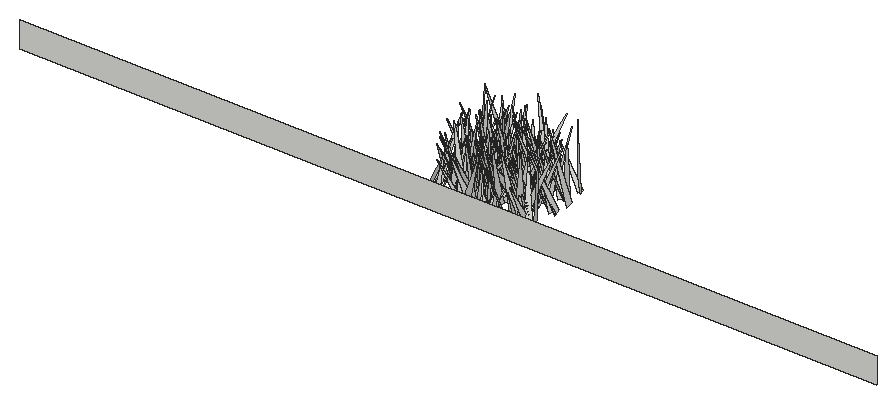
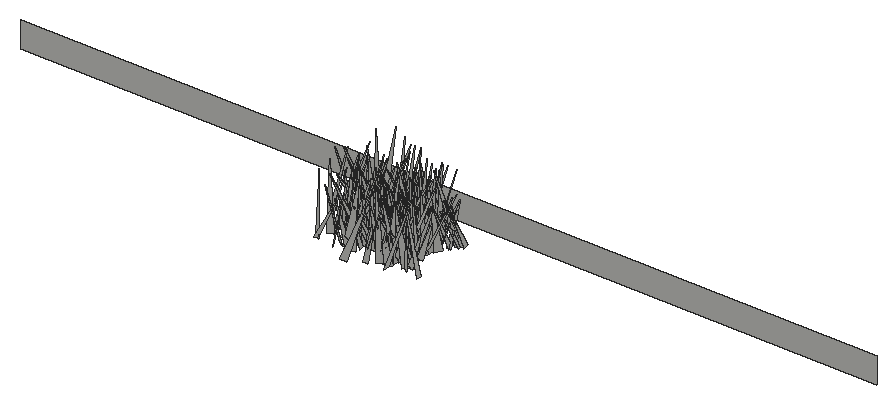
# SketchUp Ruby script. Lengths in inches.
U = 1.inch
M = Sketchup.active_model
def pt(a) = Geom::Point3d.new(a.map { |v| v * U })
def face(e, loops, mat)
  f = e.add_face(loops[0].map { |a| pt(a) })
  loops[1..].each { |l| e.add_face(l.map { |a| pt(a) }).erase! }
  f.material = f.back_material = mat if mat
  f
end
# faces: each face lists its corners as indices into pts; further lists are holes
def faces(e, pts, list, mat = nil) = list.each { |f| face(e, (f[0].is_a?(Array) ? f : [f]).map { |l| l.map { |i| pts[i] } }, mat) }
# xy, xz, yz: faces in a plane at the given z, y or x. An outline is a flat list of corners, or four numbers for a rectangle; further outlines are holes
def ring(l) = l.size == 4 ? [[l[0], l[1]], [l[2], l[1]], [l[2], l[3]], [l[0], l[3]]] : l.each_slice(2).to_a
def flat(e, list, mat, &to3) = list.each { |f| face(e, (f[0].is_a?(Array) ? f : [f]).map { |l| ring(l).map { |u, v| to3.(u, v) } }, mat) }
def xy(e, z, list, mat = nil) = flat(e, list, mat) { |x, y| [x, y, z] }
def xz(e, y, list, mat = nil) = flat(e, list, mat) { |x, z| [x, y, z] }
def yz(e, x, list, mat = nil) = flat(e, list, mat) { |y, z| [x, y, z] }
def lines(e, pts, list) = list.each { |a, b| e.add_line(pt(pts[a]), pt(pts[b])) }
# prism: a flat outline (further loops are holes) pulled along v
def prism(e, loops, v, mat = nil)
  f = face(e, loops, mat); d = Geom::Vector3d.new(v.map { |x| x * U })
  f.pushpull(f.normal.samedirection?(d) ? d.length : -d.length)
end
def box(e, o, s, mat = nil) = prism(e, [[o, [o[0] + s[0], o[1], o[2]], [o[0] + s[0], o[1] + s[1], o[2]], [o[0], o[1] + s[1], o[2]]]], [0, 0, s[2]], mat)
def at(x, y, z, deg = 0) = Geom::Transformation.translation(pt([x, y, z])) * Geom::Transformation.rotation(ORIGIN, Z_AXIS, deg.degrees)
def axes(o, x, y, z) = Geom::Transformation.new([*x, 0, *y, 0, *z, 0, *pt(o).to_a, 1])
def part(name) = M.definitions.add(name)
# library, detail: a bought-in or finely detailed component or shape, given as its bounding box
def library(name, o, s) = part(name).tap { |d| box(d.entities, o, s) }
def detail(e, o, s) = box(e.add_group.entities, o, s)
def put(e, d, t, mat = nil) = e.add_instance(d, t).tap { |i| i.material = mat if mat }
def group(e, t, mat = nil) = e.add_group.tap { |g| g.transformation = t; g.material = mat if mat }.entities
root = M.entities
c1 = part("fur_instance\#9")
p = [[0.8125,0,1.79],[0.67,-0.02,1.48],[0,-0.11,0],[0,0.11,0]]
faces(c1.entities,p,[[0,1,2,3]])
xz(root,5.77,[[0,-27.625,196.6875,-21.625]])
put(root,c1,axes([98.54,11.75,-27.1],[2.87814,-5.28951,1.31735],[-4.95416,-3.15966,-1.86304],[-2.27391,0.18887,5.72641]))
put(root,c1,axes([108.72,12.08,-27.1],[6.46231,-4.31648,2.52967],[-3.92803,-6.93665,-1.8017],[-3.09867,-0.20881,7.55958]))
put(root,c1,axes([97.8,11.71,-27.1],[2.89446,-5.47209,0.08006],[-5.31049,-2.7865,1.53693],[1.32243,0.78724,5.99662]))
put(root,c1,axes([108.44,12.38,-27.1],[4.1039,-1.37964,0.4984],[-1.03776,-3.77714,-1.91052],[-1.03675,-1.68037,3.88527]))
put(root,c1,axes([97.1,14.13,-27.1],[5.11337,-4.37567,0.02712],[-4.08728,-4.79107,-2.37351],[-1.56248,-1.78687,6.29758]))
put(root,c1,axes([110.18,13.09,-27.1],[4.14247,-2.36814,0.94959],[-1.79033,-3.98803,-2.13546],[-1.81783,-1.46881,4.26707]))
put(root,c1,axes([100.52,11.44,-27.1],[3.76138,-1.24538,0.93866],[-1.27843,-3.86595,-0.00634],[-0.89313,0.28885,3.96218]))
put(root,c1,axes([94.32,12.76,-27.1],[-3.93279,-0.23592,0.50656],[-0.05149,3.7386,1.34138],[0.55643,-1.32147,3.70448]))
put(root,c1,axes([99.45,11.81,-27.1],[1.25077,5.74635,3.18749],[6.40163,-1.79789,0.7292],[-1.48314,-2.91412,5.83551]))
put(root,c1,axes([99.67,13.3,-27.1],[6.5233,2.37968,3.04495],[3.30026,-6.53866,-1.96019],[-2.01069,-3.01183,6.66138]))
put(root,c1,axes([103.65,14.05,-27.1],[7.48346,-2.4752,1.75576],[-1.96533,-7.51292,-2.21472],[-2.31232,-1.62508,7.56464]))
put(root,c1,axes([104.87,12.96,-27.1],[-1.89303,-4.40404,0.51291],[-4.43222,1.86471,-0.34716],[-0.11875,0.60786,4.78107]))
put(root,c1,axes([103.4,14.22,-27.1],[-5.97447,-2.65496,2.2585],[-2.10106,6.3191,1.8704],[2.78122,-0.92951,6.26456]))
put(root,c1,axes([107.73,14.55,-27.1],[5.80631,-5.6916,0.53269],[-5.68589,-5.82856,-0.29992],[-0.59055,0.15799,8.12513]))
put(root,c1,axes([103.21,11.5,-27.1],[-0.85161,3.55792,0.87868],[3.50079,1.05663,-0.88551],[1.08413,-0.61714,3.54963]))
put(root,c1,axes([103.73,12.08,-27.1],[3.9323,-0.29865,1.47953],[-0.48436,-4.16008,0.44758],[-1.42954,0.58799,3.91814]))
put(root,c1,axes([96.6,12.32,-27.1],[5.34271,-3.44394,4.19103],[-3.85612,-6.54857,-0.46545],[-3.8152,1.796,6.33945]))
put(root,c1,axes([100.63,11.89,-27.1],[-2.63101,2.88231,1.12737],[2.88894,2.81797,-0.46255],[1.11028,-0.50218,3.87505]))
put(root,c1,axes([101.61,15.49,-27.1],[-1.56855,-7.63886,0.47282],[-7.63369,1.59619,0.46371],[0.55001,0.36889,7.78444]))
put(root,c1,axes([101.04,15.37,-27.1],[-1.24529,-7.71146,0.7872],[-7.61167,1.36728,1.35282],[1.46589,0.54863,7.69333]))
put(root,c1,axes([103.93,12.45,-27.1],[-0.42673,3.51272,1.26133],[3.73148,0.37463,0.21911],[-0.0791,-1.27778,3.53176]))
put(root,c1,axes([93.95,15.29,-27.1],[-5.87667,-3.9224,1.1719],[-3.54254,5.90008,1.98324],[2.05159,-1.04767,6.78139]))
put(root,c1,axes([104.39,17.625,-27.1],[6.48177,-5.01878,0.45242],[-4.24735,-5.8379,-3.90962],[-2.71162,-2.85253,7.2053]))
put(root,c1,axes([90.46,12.68,-27.1],[1.50954,-3.07856,1.78204],[-3.55315,-1.39659,0.59714],[-0.16832,1.87187,3.37633]))
put(root,c1,axes([103.32,12.72,-27.1],[4.26257,2.91433,0.00484],[2.86478,-4.18851,-0.95515],[0.53516,-0.79116,5.0745]))
put(root,c1,axes([101.18,13.5,-27.1],[-4.07281,-4.5818,0.7427],[-4.55178,3.7491,-1.83244],[-0.90871,1.75604,5.85003]))
put(root,c1,axes([110.46,13.58,-27.1],[-2.82559,-5.19892,1.36333],[-5.31081,2.46391,-1.61114],[-0.82624,1.9421,5.69358]))
put(root,c1,axes([101.12,13.64,-27.1],[-2.2184,-4.85625,2.50772],[-5.03427,2.86928,1.10295],[2.1279,1.72546,5.22379]))
put(root,c1,axes([91.81,12.22,-27.1],[4.67763,2.46387,0.32375],[2.42875,-4.67875,0.51598],[-0.52599,0.30722,5.26162]))
put(root,c1,axes([96.28,12.86,-27.1],[3.51282,6.48869,2.15536],[6.79895,-3.57131,-0.32959],[-0.72316,-2.057,7.37118]))
put(root,c1,axes([101.98,16.15,-27.1],[0.91658,-6.09487,0.23316],[-5.96683,-0.94489,-1.24341],[-1.26442,0.04079,6.03668]))
put(root,c1,axes([112.29,13.32,-27.1],[-4.83531,-1.63891,2.39644],[-2.01972,5.24312,-0.48946],[2.08559,1.27782,5.08199]))
put(root,c1,axes([93.04,14.27,-27.1],[-5.61419,2.77509,3.47904],[3.15086,6.4338,-0.04739],[3.14276,-1.49299,6.26243]))
put(root,c1,axes([94.93,15.09,-27.1],[-3.76268,-4.24685,0.11424],[-4.17448,3.66755,-1.15295],[-0.78896,0.84846,5.55555]))
put(root,c1,axes([88.44,13.02,-27.1],[5.14686,-0.10254,0.48257],[-0.21946,-5.00543,1.27711],[-0.44184,1.29176,4.98695]))
put(root,c1,axes([90.48,15.46,-27.1],[-0.08561,-4.51883,0.61864],[-4.55746,0.06047,-0.18896],[-0.17898,0.62161,4.51569]))
put(root,c1,axes([100.42,13.8125,-27.1],[-4.38445,3.57185,1.79964],[3.76738,4.58485,0.07863],[1.34299,-1.20052,5.65467]))
put(root,c1,axes([109.75,12.12,-27.1],[-6.16922,0.32467,1.04524],[-0.06119,5.87189,-2.18505],[1.09279,2.16166,5.77844]))
put(root,c1,axes([100.8125,13.96,-27.1],[-6.07164,-2.28107,2.04855],[-2.55827,6.27412,-0.5961],[1.68971,1.3026,6.45854]))
put(root,c1,axes([98.98,15.98,-27.1],[-1.13114,-4.608,0.05517],[-4.59723,1.12439,-0.34274],[-0.31976,0.13515,4.73241]))
put(root,c1,axes([98.36,14.21,-27.1],[4.34126,2.62004,0.01209],[2.52851,-4.18338,-1.34808],[0.68659,-1.1602,4.88813]))
put(root,c1,axes([98.34,13.66,-27.1],[4.70359,-4.43483,0.77561],[-4.1988,-3.91632,3.07011],[1.62462,2.71804,5.6891]))
put(root,c1,axes([110.84,12.96,-27.1],[-3.10471,5.12305,0.88051],[5.18598,3.12286,0.11631],[0.35573,-0.81381,5.98927]))
put(root,c1,axes([97.03,15.39,-27.1],[-4.89402,-3.33819,1.83703],[-3.30827,5.20635,0.64726],[1.89038,0.46913,5.88863]))
put(root,c1,axes([108.12,16.37,-27.1],[-3.94207,-4.94022,1.13908],[-4.81769,4.09962,1.10733],[1.57897,0.1748,6.2225]))
put(root,c1,axes([93.34,14.85,-27.1],[3.78435,-1.32179,0.68035],[-1.35222,-3.83372,0.07338],[-0.61764,0.29457,4.00787]))
put(root,c1,axes([100.32,14.03,-27.1],[-1.02594,6.32348,2.52203],[6.58274,1.57191,-1.26344],[1.73626,-2.22313,6.28034]))
put(root,c1,axes([99.11,15.625,-27.1],[1.24719,-3.91493,0.4967],[-3.8954,-1.13791,0.81231],[0.63182,0.71228,4.02769]))
put(root,c1,axes([100.35,15.59,-27.1],[-1.33091,-4.34516,1.37723],[-4.35803,1.6335,0.94222],[1.33595,0.99989,4.44566]))
put(root,c1,axes([93.37,14.92,-27.1],[0.69074,-4.72184,2.34998],[-4.89788,-1.45354,-1.48096],[-1.95676,1.97148,4.53648]))
put(root,c1,axes([89.04,13.88,-27.1],[4.0967,-0.1052,0.02727],[-0.10864,-3.93802,1.12914],[0.00278,1.12946,3.93942]))
put(root,c1,axes([94.33,14.38,-27.1],[-2.33068,3.85921,0.35584],[3.66264,2.05758,1.6744],[-1.26695,-1.15111,4.18592]))
put(root,c1,axes([89.42,13.98,-27.1],[0.24663,7.62872,2.41582],[7.70784,0.42293,-2.12242],[2.15005,-2.39126,7.33168]))
put(root,c1,axes([104.46,16.01,-27.1],[-2.38494,-6.16406,1.52656],[-6.35023,2.30898,-0.59758],[-0.0234,1.63919,6.58229]))
put(root,c1,axes([108.95,14.06,-27.1],[5.79439,-3.93356,1.43708],[-4.17619,-5.2444,2.48372],[0.31237,2.85246,6.54821]))
put(root,c1,axes([92.67,14.32,-27.1],[-3.84784,-1.19504,0.32807],[-1.23606,3.62421,-1.29571],[-0.08892,1.33363,3.81512]))
put(root,c1,axes([106.33,16.25,-27.1],[-3.36385,-0.86607,1.07357],[-0.51946,3.41676,1.12873],[1.27781,-0.89095,3.28504]))
put(root,c1,axes([103.16,15.92,-27.1],[-3.34237,-3.67886,0.49489],[-3.71061,3.29315,-0.58039],[-0.10119,0.75599,4.93646]))
put(root,c1,axes([91.96,16.72,-27.1],[-3.17916,-2.57933,0.00353],[-2.53731,3.12837,0.73174],[0.46373,-0.56605,4.02798]))
put(root,c1,axes([105.08,15.55,-27.1],[-3.3946,-3.12525,1.18102],[-3.29173,3.41661,-0.4203],[0.5714,1.11577,4.59499]))
put(root,c1,axes([105.97,17.65,-27.1],[2.24091,-5.47361,0.67385],[-5.23088,-2.33999,-1.61199],[-1.7471,-0.01469,5.69066]))
put(root,c1,axes([98.25,15.02,-27.1],[4.49912,0.07902,0.02983],[0.07502,-4.46879,0.52292],[-0.03881,0.52233,4.46932]))
put(root,c1,axes([97.99,16.47,-27.1],[1.8485,-3.49978,1.33816],[-3.45042,-2.17169,-0.91344],[-1.46071,0.70098,3.8511]))
put(root,c1,axes([110.15,19.25,-27.1],[-3.50557,-5.51536,0.11612],[-4.95597,3.20905,2.80393],[2.42302,-1.41579,5.90306]))
put(root,c1,axes([106.26,16.66,-27.1],[2.2039,-6.87435,1.74953],[-7.02125,-1.85328,1.56272],[1.00974,2.1174,7.04782]))
put(root,c1,axes([103.87,15.71,-27.1],[-0.77186,4.35622,1.72795],[4.2436,-0.09339,2.13104],[-1.98854,-1.8902,3.87699]))
put(root,c1,axes([113.22,18.26,-27.1],[-7.42684,-1.75978,1.28146],[-1.36577,7.3143,2.12899],[1.69519,-1.81689,7.32954]))
put(root,c1,axes([109.69,16.92,-27.1],[-5.35424,-1.86738,0.02315],[-1.86377,5.3475,0.29345],[0.11847,-0.26947,5.66294]))
put(root,c1,axes([95.07,18.68,-27.1],[7.37439,-3.31849,1.28024],[-2.90244,-7.31769,-2.24953],[-2.05603,-1.57231,7.76747]))
put(root,c1,axes([102.41,13.9,-27.1],[0.90469,6.24799,0.05202],[5.52251,-0.775,-2.9597],[2.92267,-0.46962,5.57638]))
put(root,c1,axes([95.3,13.15,-27.1],[-7.34828,2.49323,1.09592],[2.03506,7.1224,-2.5582],[1.80991,2.11416,7.32591]))
put(root,c1,axes([97.38,17.34,-27.1],[2.10827,-4.41232,0.88185],[-4.4927,-2.11805,0.1432],[-0.24874,0.85808,4.88803]))
put(root,c1,axes([101.06,16,-27.1],[1.63148,3.88333,0.8996],[3.80186,-1.22375,-1.61232],[1.19808,-1.40479,3.89132]))
put(root,c1,axes([107.17,18.27,-27.1],[1.92624,-6.27783,0.49509],[-6.26935,-1.863,0.76884],[0.59288,0.69623,6.52153]))
put(root,c1,axes([101.15,19.08,-27.1],[5.45875,-2.61976,0.1584],[-2.41646,-5.15945,-2.05595],[-1.02417,-1.78972,5.6951]))
put(root,c1,axes([104.25,19.42,-27.1],[-5.79035,-4.99721,0.36352],[-4.82955,5.71454,1.62848],[1.33407,-1.00217,7.47317]))
put(root,c1,axes([93.13,18.07,-27.1],[2.46891,-7.20313,1.70316],[-7.36136,-2.57683,-0.22704],[-0.77207,1.53499,7.61111]))
put(root,c1,axes([92.8,15.74,-27.1],[3.62084,3.81527,1.03017],[3.87963,-3.69771,0.05854],[-0.75237,-0.70613,5.25959]))
put(root,c1,axes([105.57,16.87,-27.1],[3.73995,-4.97965,1.07609],[-4.97131,-3.27521,2.12161],[1.114,2.10195,5.85517]))
put(root,c1,axes([90.45,15.07,-27.1],[4.99403,0.89918,1.35491],[0.3935,-4.91429,1.81096],[-1.5778,1.62046,4.74018]))
put(root,c1,axes([95.3125,15.46,-27.1],[4.61387,-2.10989,0.31356],[-1.93342,-3.82099,2.73855],[0.90102,2.60502,4.2708]))
put(root,c1,axes([96.03,16.4,-27.1],[3.36091,-1.13304,0.9234],[-1.35023,-3.29337,0.87337],[-0.55977,1.1411,3.43755]))
put(root,c1,axes([94.78,18.22,-27.1],[-2.52034,-4.28654,0.32351],[-4.12689,2.30776,-1.57296],[-1.20326,1.06349,4.71724]))
put(root,c1,axes([113.24,18.05,-27.1],[-6.30191,-3.29477,0.26908],[-3.30318,6.25333,-0.79169],[-0.13009,0.82599,7.06702]))
put(root,c1,axes([98.65,18.3125,-27.1],[-4.19066,-2.50752,1.09961],[-2.47633,4.32875,0.43379],[1.16817,0.18082,4.86427]))
put(root,c1,axes([112.28,17.91,-27.1],[-4.9541,1.83691,1.27432],[2.05779,4.95762,0.85363],[0.87385,-1.26054,5.21428]))
put(root,c1,axes([102.53,14.22,-27.1],[3.62911,6.60842,0.2466],[6.35712,-3.56375,1.94657],[-1.82181,0.72867,7.28371]))
put(root,c1,axes([91.14,17.54,-27.1],[5.12672,-4.5376,2.59386],[-5.0883,-5.16347,1.02416],[-1.19461,2.5199,6.76936]))
put(root,c1,axes([98.95,19.43,-27.1],[-3.68425,-5.36529,0.32526],[-5.32374,3.58793,-1.11818],[-0.74155,0.8979,6.41168]))
put(root,c1,axes([103.25,18.7,-27.1],[-1.22069,-3.41408,1.05948],[-3.55821,1.26785,-0.01408],[0.34288,1.00256,3.62571]))
put(root,c1,axes([99.66,18.9375,-27.1],[-3.20699,2.34244,2.63387],[2.95903,3.72406,0.29089],[1.91533,-1.83124,3.96071]))
put(root,c1,axes([108.55,18.625,-27.1],[4.54413,5.8348,1.67226],[5.93472,-3.83302,-2.75273],[1.27295,-2.95864,6.86415]))
put(root,c1,axes([103.3125,18.64,-27.1],[-0.92871,-3.83483,1.6083],[-4.04735,1.2119,0.55253],[0.95473,1.40727,3.90681]))
put(root,c1,axes([96.76,18.89,-27.1],[0.02782,-4.7345,1.86898],[-5.06027,0.17616,0.52158],[0.54982,1.86087,4.70577]))
put(root,c1,axes([108.96,19.18,-27.1],[3.6892,-1.49713,1.29137],[-1.47127,-3.90506,-0.32413],[-1.32076,0.16824,3.96818]))
put(root,c1,axes([92.43,20.0625,-27.1],[2.19919,-5.46865,1.19281],[-5.58851,-2.07385,0.79564],[0.31218,1.39943,5.84033]))
put(root,c1,axes([92.4,20.07,-27.1],[-5.87087,-0.65311,0.1721],[-0.62527,5.82501,0.77566],[0.25536,-0.75237,5.85594]))
put(root,c1,axes([104.39,17.93,-27.1],[3.12045,6.97557,0.92804],[6.87353,-2.80376,-2.03727],[1.5081,-1.6545,7.36514]))
put(root,c1,axes([110.32,14.52,-27.1],[5.94606,5.36025,0.59468],[4.2161,-5.17199,4.4628],[-3.36309,2.9933,6.64615]))
put(root,c1,axes([92,18.89,-27.1],[-5.13165,1.21269,1.54361],[1.09048,5.35359,-0.58061],[1.63224,0.23592,5.24093]))
put(root,c1,axes([106.85,20.65,-27.1],[2.3512,-5.85332,1.44977],[-6.03015,-2.28819,0.5412],[-0.02311,1.54732,6.28463]))
put(root,c1,axes([100.87,20.15,-27.1],[4.61711,2.95667,1.94744],[3.35791,-4.67134,-0.86895],[-1.12198,-1.8135,5.41336]))
put(root,c1,axes([99.21,19.03,-27.1],[-3.06534,4.86368,0.18481],[4.51167,2.75744,2.26433],[-1.82603,-1.35165,5.28436]))
put(root,c1,axes([101.11,20.35,-27.1],[4.30698,0.82715,0.77594],[0.97071,-4.26434,-0.84231],[-0.5865,-0.98365,4.30404]))
put(root,c1,axes([100.98,20.16,-27.1],[-2.4507,-4.58404,1.24543],[-4.71435,2.17524,-1.27033],[-0.58261,1.68089,5.0404]))
put(root,c1,axes([106.03,20.35,-27.1],[4.89735,3.35239,2.18214],[3.80193,-4.97328,-0.89225],[-1.24321,-2.00306,5.86741]))
put(root,c1,axes([104.77,18.31,-27.1],[1.00631,5.78428,1.17144],[5.41169,-1.37849,2.15781],[-2.35451,-0.6962,5.46025]))
put(root,c1,axes([94.97,21.88,-27.1],[-4.99858,-6.00178,0.67378],[-6.03784,4.94565,-0.739],[-0.1407,0.9901,7.77567]))
put(root,c1,axes([106.64,22.57,-27.1],[-7.7703,-1.5883,1.42664],[-1.2052,7.70803,2.01725],[1.76224,-1.7318,7.67014]))
put(root,c1,axes([93.95,20.4,-27.1],[-5.48132,1.03762,0.48302],[1.07413,5.47965,0.41785],[0.39525,-0.50168,5.563]))
put(root,c1,axes([94.95,20.97,-27.1],[5.5976,-0.64404,1.05715],[-0.59203,-5.69245,-0.3332],[-1.08713,-0.21617,5.62467]))
put(root,c1,axes([93.49,22.07,-27.1],[0.81031,-5.69395,0.84212],[-5.55553,-0.55126,1.61834],[1.50543,1.03047,5.51893]))
put(root,c1,axes([110.77,22.91,-27.1],[-3.23676,-6.95107,0.75182],[-6.9834,3.25434,0.02332],[0.33861,0.67166,7.66769]))
put(root,c1,axes([93.72,21.75,-27.1],[-0.85908,-3.57953,0.71794],[-3.54097,0.99653,0.73143],[0.88884,0.51028,3.60778]))
put(root,c1,axes([99.27,20.74,-27.1],[-4.79619,2.23097,0.90337],[2.34699,4.78153,0.65218],[0.53379,-0.97799,5.24932]))
put(root,c1,axes([113.23,21.92,-27.1],[-7.82049,-1.65264,1.82204],[-1.48703,8.01344,0.88582],[1.95953,-0.51451,7.94397]))
put(root,c1,axes([94.43,22.45,-27.1],[6.50516,0.09741,3.11354],[0.81371,-7.01185,-1.48071],[-3.00691,-1.68675,6.33514]))
put(root,c1,axes([104.8125,20.66,-27.1],[3.28542,-2.52777,1.83261],[-2.97263,-3.34603,0.71392],[-0.95477,1.71946,4.08337]))
put(root,c1,axes([93.3125,21.35,-27.1],[6.93717,-2.75986,2.51351],[-2.97128,-7.29338,0.19237],[-2.25967,1.11744,7.46352]))
put(root,c1,axes([102.1,21.9,-27.1],[1.8151,-3.86013,1.55176],[-3.9232,-2.15155,-0.76319],[-1.38458,1.03602,4.19675]))
put(root,c1,axes([100.08,19.92,-27.1],[3.50829,2.33455,0.59392],[2.17247,-3.51961,1.00185],[-1.04078,0.52272,4.09323]))
put(root,c1,axes([100.59,19.74,-27.1],[-4.5545,1.12209,0.15618],[1.0267,4.36161,-1.39615],[0.47894,1.3207,4.4781]))
put(root,c1,axes([97.65,24.4,-27.1],[7.10031,-2.91459,1.55919],[-2.29482,-7.00551,-2.64516],[-2.37902,-1.94118,7.20502]))
put(root,c1,axes([100.1875,20.67,-27.1],[-4.76219,-1.42096,1.84075],[-1.91994,4.76946,-1.2853],[1.31199,1.82182,4.80058]))
put(root,c1,axes([112.125,23,-27.1],[-3.86878,-4.9807,0.99535],[-5.05831,3.89149,-0.18804],[0.45997,0.9025,6.30392]))
put(root,c1,axes([108.9,21.53,-27.1],[4.04203,-2.33275,1.48439],[-2.65208,-4.01454,0.91276],[-0.78205,1.55722,4.57675]))
put(root,c1,axes([99.34,22.06,-27.1],[-3.99444,1.28958,0.25526],[1.31279,3.95594,0.55757],[0.06915,-0.60932,4.16025]))
put(root,c1,axes([91.93,21.95,-27.1],[-2.38269,3.95567,1.05235],[4.03891,2.07425,1.34786],[-0.66484,-1.57548,4.41677]))
put(root,c1,axes([107.99,24.28,-27.1],[3.38324,-1.277,0.34003],[-0.90165,-2.91389,-1.97203],[-0.96612,-1.75247,3.03119]))
put(root,c1,axes([98.84,22.26,-27.1],[-5.61783,-2.93903,2.21928],[-3.25584,5.85535,-0.48739],[1.72124,1.48327,6.32142]))
put(root,c1,axes([98.36,23.65,-27.1],[1.13187,-5.42392,1.09616],[-5.52646,-1.05128,0.50466],[0.2806,1.17367,5.51773]))
put(root,c1,axes([98.62,21.43,-27.1],[-5.41908,-0.82486,1.13145],[-1.12996,5.24719,-1.58656],[0.82691,1.76453,5.24687]))
put(root,c1,axes([106.2,22.67,-27.1],[-3.46887,0.5768,0.94943],[0.60796,3.5911,0.03958],[0.92978,-0.19616,3.51628]))
put(root,c1,axes([110.52,24.38,-27.1],[1.17808,-6.7396,1.1437],[-6.76699,-0.98532,1.16408],[0.96855,1.31342,6.74203]))
put(root,c1,axes([110.67,22.69,-27.1],[-3.89894,3.87426,1.21258],[4.05705,3.77806,0.97396],[0.14352,-1.54866,5.40953]))
put(root,c1,axes([109.18,20.91,-27.1],[-7.08431,2.74004,0.68893],[2.60293,7.0529,-1.28499],[1.09872,0.95845,7.48626]))
put(root,c1,axes([96.21,22.5,-27.1],[6.43486,-0.85229,1.84553],[-1.08084,-6.62327,0.70985],[-1.72168,0.97247,6.45212]))
put(root,c1,axes([97.52,22.48,-27.1],[-3.69275,-0.52533,1.17947],[-0.76187,3.77166,-0.70545],[1.04243,0.89562,3.66261]))
put(root,c1,axes([93.67,24.68,-27.1],[3.36896,-5.0045,1.18358],[-5.04079,-3.49374,-0.42432],[-1.01802,0.73793,6.01788]))
put(root,c1,axes([92.1,21.97,-27.1],[4.14579,-2.60609,2.17076],[-3.31381,-3.84297,1.71517],[-0.72292,2.67047,4.58667]))
put(root,c1,axes([95.92,24.14,-27.1],[-2.42816,-5.42807,1.43938],[-5.61543,2.33238,-0.67728],[-0.05217,1.5899,5.90772]))
put(root,c1,axes([92.36,22.12,-27.1],[-7.10447,-2.39928,3.44832],[-3.25719,7.42464,-1.54476],[2.65295,2.69055,7.33783]))
put(root,c1,axes([96.46,22.5,-27.1],[-4.11869,2.39634,0.55767],[2.352,4.15398,-0.47915],[0.72219,0.13795,4.74094]))
put(root,c1,axes([93.34,23.48,-27.1],[7.44021,-1.05618,0.97458],[-1.13327,-7.472,0.55406],[-0.88376,0.68976,7.49435]))
put(root,c1,axes([105.98,24.64,-27.1],[-1.13695,-6.80591,1.9758],[-6.92615,0.64332,-1.76957],[-1.50086,2.18691,6.66945]))
put(root,c1,axes([98,22.96,-27.1],[-3.61656,3.24074,0.55892],[3.26072,3.64166,-0.01623],[0.42715,-0.36083,4.85609]))
put(root,c1,axes([94.75,25.36,-27.1],[-5.48359,2.23586,1.70204],[2.68404,5.27249,1.72124],[0.83185,-2.27324,5.66623]))
put(root,c1,axes([105.73,25.33,-27.1],[2.79472,-2.37927,0.19168],[-2.37504,-2.80125,-0.14262],[-0.23842,0.01542,3.66757]))
put(root,c1,axes([98.94,25.44,-27.1],[-4.40075,-1.21691,1.44212],[-0.98766,4.60363,0.87078],[1.60783,-0.50284,4.4821]))
put(root,c1,axes([95.34,23.27,-27.1],[-1.64071,6.20292,1.41522],[6.35653,1.66047,0.09149],[0.27128,-1.39198,6.41559]))
put(root,c1,axes([91.86,25.91,-27.1],[3.71453,-6.09838,0.78607],[-6.05056,-3.46164,1.73599],[1.09493,1.55972,6.92635]))
put(root,c1,axes([101.55,25.42,-27.1],[-4.35453,-4.53446,2.05004],[-4.74623,4.60317,0.10013],[1.49574,1.4055,6.28595]))
put(root,c1,axes([103.41,23.99,-27.1],[-5.08391,3.17186,1.29588],[3.17676,5.23223,-0.34381],[1.28383,-0.38638,5.98237]))
put(root,c1,axes([102.27,23.66,-27.1],[-6.74391,-2.32387,0.77011],[-2.44649,6.31426,-2.37034],[-0.09,2.49068,6.72772]))
put(root,c1,axes([106.95,24.99,-27.1],[-6.4254,-4.61842,2.37343],[-5.01235,6.50279,-0.91585],[1.35622,2.15235,7.85982]))
put(root,c1,axes([96.59,21.8,-27.1],[-4.56686,4.07542,0.09193],[3.68922,4.19072,-2.51023],[1.73411,1.8173,5.58247]))
put(root,c1,axes([98.3,23.55,-27.1],[-2.89622,3.26829,0.45856],[3.08153,2.89643,-1.18106],[1.18158,0.4572,4.20415]))
put(root,c1,axes([101.58,22.89,-27.1],[-1.51981,5.35977,0.02073],[5.22969,1.48762,-1.21441],[1.17387,0.31183,5.43711]))
put(root,c1,axes([100.94,24.48,-27.1],[-0.82841,6.75025,1.93378],[7.00258,0.65031,0.72978],[-0.51887,-2.00072,6.76162]))
put(root,c1,axes([94.92,26.58,-27.1],[4.55576,-0.64185,1.19418],[-0.37344,-4.61891,-1.05794],[-1.3033,-0.92017,4.47746]))
put(root,c1,axes([104.77,24.61,-27.1],[-1.73609,5.26171,0.91511],[5.1615,1.40586,1.70864],[-1.37182,-1.3693,5.27069]))
put(root,c1,axes([94.49,25.68,-27.1],[5.43956,-0.0104,1.6458],[0.01524,-5.68242,-0.08629],[-1.64576,-0.087,5.43889]))
put(root,c1,axes([104.83,27.3,-27.1],[-2.5051,-3.46967,0.23869],[-3.39401,2.50314,0.76559],[0.75915,-0.25846,4.21047]))
put(root,c1,axes([104.36,27.56,-27.1],[-1.56968,-5.60909,0.11931],[-5.50885,1.51747,-1.1357],[-1.06238,0.41882,5.71278]))
put(root,c1,axes([87.98,27.12,-27.1],[8.03575,1.73258,0.69022],[1.85682,-7.7181,-2.24381],[-0.17451,-2.34107,7.90825]))
put(root,c1,axes([91.3,25.53,-27.1],[-1.35537,3.98703,1.26023],[4.07237,0.95801,1.34893],[-0.94888,-1.58348,3.98921]))
put(root,c1,axes([96.74,24.37,-27.1],[-5.17368,4.83178,0.63052],[4.85594,5.1888,0.08232],[0.40437,-0.49072,7.07858]))
put(root,c1,axes([102.85,24.18,-27.1],[1.48421,7.77893,1.22221],[7.56365,-1.06243,-2.42301],[2.19017,-1.60247,7.53948]))
put(root,c1,axes([94.6,27.43,-27.1],[3.61715,-5.66391,0.01487],[-5.50634,-3.51236,1.58351],[1.3268,0.86448,6.53117]))
put(root,c1,axes([103.3,27.12,-27.1],[2.16413,-4.87719,1.14426],[-4.95965,-2.26151,-0.2591],[-0.70577,0.93721,5.32947]))
put(root,c1,axes([102.84,25.23,-27.1],[4.75143,0.92242,1.33841],[0.70934,-4.89704,0.85681],[-1.46255,0.62163,4.7637]))
put(root,c1,axes([96.75,27.49,-27.1],[1.17018,-6.95871,1.51726],[-7.0392,-0.89595,1.31981],[1.08411,1.69372,6.93189]))
put(root,c1,axes([99.89,23.58,-27.1],[-6.30964,2.41528,1.06239],[1.96226,6.1361,-2.29599],[1.76402,1.81341,6.35402]))
put(root,c1,axes([96.51,27.07,-27.1],[-2.7828,-3.97435,1.2381],[-4.07565,2.90431,0.16237],[0.84701,0.91751,4.84903]))
put(root,c1,axes([95.79,24.53,-27.1],[0.08321,7.29137,1.2347],[7.39423,-0.10178,0.10277],[-0.11831,-1.23331,7.29112]))
put(root,c1,axes([97.23,26.63,-27.1],[-3.6032,0.74818,1.09352],[0.87855,3.72087,0.34907],[0.99182,-0.57787,3.66346]))
put(root,c1,axes([91.48,26.59,-27.1],[-1.7362,-3.80786,1.79903],[-4.13168,1.91701,0.07019],[0.81577,1.60498,4.18441]))
put(root,c1,axes([98.87,28.88,-27.1],[-0.42981,-6.03201,0.26249],[-6.01913,0.44871,0.45551],[0.47339,0.22867,6.03012]))
put(root,c1,axes([111.65,27.05,-27.1],[-4.58774,2.19144,0.09862],[2.15217,4.45217,1.18567],[-0.42461,-1.11142,4.94408]))
put(root,c1,axes([106.79,26.07,-27.1],[3.4607,5.10853,1.2476],[5.25066,-3.43918,-0.48234],[-0.29016,-1.30574,6.15149]))
put(root,c1,axes([107.4375,27.4,-27.1],[-4.91949,-2.25789,1.34677],[-2.33985,5.06309,-0.05864],[1.19873,0.61667,5.41258]))
put(root,c1,axes([111.65,26.74,-27.1],[-3.98091,-5.38333,3.048],[-6.04161,4.16252,-0.53901],[1.33021,2.79489,6.67363]))
put(root,c1,axes([104.03,27.29,-27.1],[3.98681,-3.04122,0.56389],[-3.08769,-3.85909,1.01744],[0.18196,1.14894,4.91004]))
put(root,c1,axes([94.67,28.25,-27.1],[-7.8071,-1.03462,1.04066],[-0.93299,7.84786,0.80297],[1.13267,-0.66693,7.83431]))
put(root,c1,axes([102.57,30.55,-27.1],[3.27442,-5.47757,0.11686],[-5.10679,-3.10069,-2.24625],[-1.98447,-1.05885,5.97327]))
put(root,c1,axes([104.73,26.61,-27.1],[-3.07753,7.46975,2.03134],[7.70521,2.74591,1.57617],[-0.74375,-2.46119,7.92363]))
